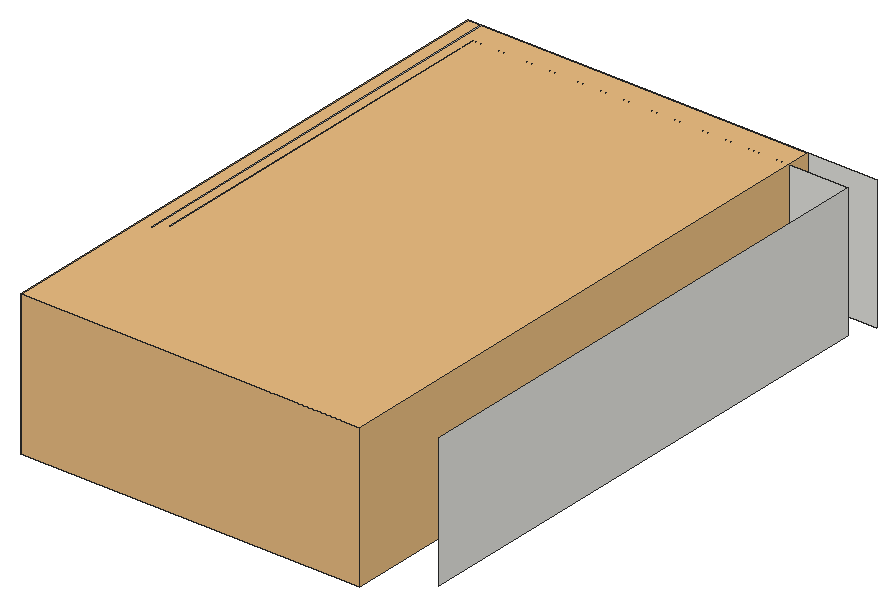
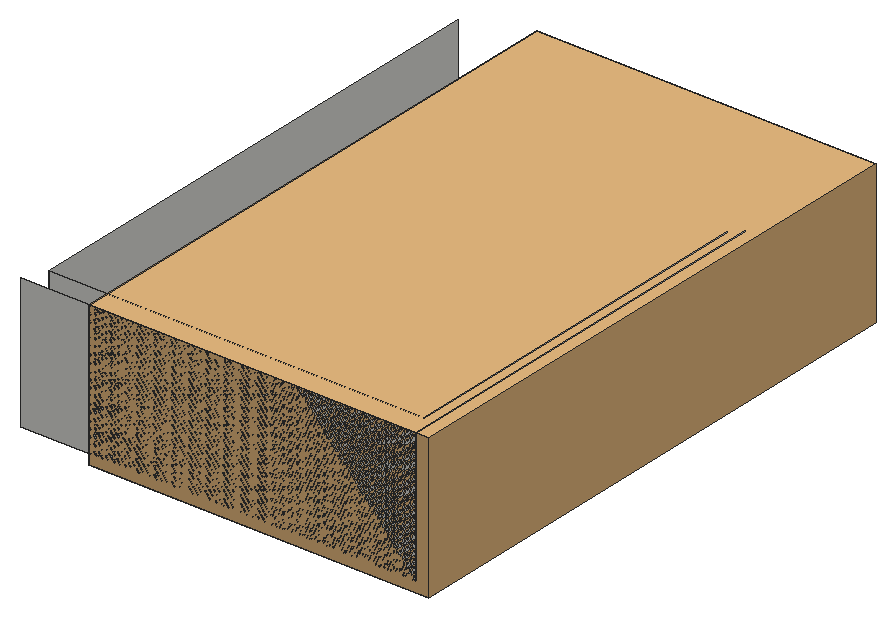
# SketchUp Ruby script. Lengths in inches.
U = 1.inch
M = Sketchup.active_model
def pt(a) = Geom::Point3d.new(a.map { |v| v * U })
def face(e, loops, mat)
  f = e.add_face(loops[0].map { |a| pt(a) })
  loops[1..].each { |l| e.add_face(l.map { |a| pt(a) }).erase! }
  f.material = f.back_material = mat if mat
  f
end
# faces: each face lists its corners as indices into pts; further lists are holes
def faces(e, pts, list, mat = nil) = list.each { |f| face(e, (f[0].is_a?(Array) ? f : [f]).map { |l| l.map { |i| pts[i] } }, mat) }
# xy, xz, yz: faces in a plane at the given z, y or x. An outline is a flat list of corners, or four numbers for a rectangle; further outlines are holes
def ring(l) = l.size == 4 ? [[l[0], l[1]], [l[2], l[1]], [l[2], l[3]], [l[0], l[3]]] : l.each_slice(2).to_a
def flat(e, list, mat, &to3) = list.each { |f| face(e, (f[0].is_a?(Array) ? f : [f]).map { |l| ring(l).map { |u, v| to3.(u, v) } }, mat) }
def xy(e, z, list, mat = nil) = flat(e, list, mat) { |x, y| [x, y, z] }
def xz(e, y, list, mat = nil) = flat(e, list, mat) { |x, z| [x, y, z] }
def yz(e, x, list, mat = nil) = flat(e, list, mat) { |y, z| [x, y, z] }
def lines(e, pts, list) = list.each { |a, b| e.add_line(pt(pts[a]), pt(pts[b])) }
# prism: a flat outline (further loops are holes) pulled along v
def prism(e, loops, v, mat = nil)
  f = face(e, loops, mat); d = Geom::Vector3d.new(v.map { |x| x * U })
  f.pushpull(f.normal.samedirection?(d) ? d.length : -d.length)
end
def box(e, o, s, mat = nil) = prism(e, [[o, [o[0] + s[0], o[1], o[2]], [o[0] + s[0], o[1] + s[1], o[2]], [o[0], o[1] + s[1], o[2]]]], [0, 0, s[2]], mat)
def at(x, y, z, deg = 0) = Geom::Transformation.translation(pt([x, y, z])) * Geom::Transformation.rotation(ORIGIN, Z_AXIS, deg.degrees)
def axes(o, x, y, z) = Geom::Transformation.new([*x, 0, *y, 0, *z, 0, *pt(o).to_a, 1])
def part(name) = M.definitions.add(name)
# library, detail: a bought-in or finely detailed component or shape, given as its bounding box
def library(name, o, s) = part(name).tap { |d| box(d.entities, o, s) }
def detail(e, o, s) = box(e.add_group.entities, o, s)
def put(e, d, t, mat = nil) = e.add_instance(d, t).tap { |i| i.material = mat if mat }
def group(e, t, mat = nil) = e.add_group.tap { |g| g.transformation = t; g.material = mat if mat }.entities
root = M.entities
M.materials.add("1122 AP 7994 PEACH ROSE").color = [254, 227, 201]
M.materials.add("[Quartz Light Grey]").color = [251, 251, 252]
c1 = library("Group\#12",[-2,-2,0],[309,506,129])
xy(root,152.82,[[40.86,300.07,40.7,300.09,40.55,300.11,40.47,300.12,40.39,300.14,40.32,300.15,40.16,300.19,40.09,300.22,40.01,300.24,39.8,300.33,39.72,300.36,39.65,300.4,39.58,300.43,39.52,300.47,39.38,300.55,39.32,300.6,39.25,300.64,38.95,300.89,38.89,300.95,38.84,301.01,38.79,301.0625,38.74,301.12,38.68,301.18,38.64,301.24,38.59,301.31,38.54,301.37,38.5,301.4375,38.46,301.5,38.34,301.71,38.28,301.85,38.24,301.92,38.22,302,38.1875,302.07,38.16,302.14,38.14,302.22,38.12,302.29,38.08,302.45,38.07,302.52,38.05,302.6,38.03,302.76,38.03,302.84,38.02,302.91,38.02,303.23,38.03,303.31,38.03,303.38,38.05,303.54,38.07,303.62,38.08,303.69,38.12,303.85,38.14,303.92,38.16,304,38.1875,304.07,38.22,304.15,38.24,304.22,38.28,304.29,38.34,304.43,38.46,304.64,38.5,304.7,38.54,304.77,38.59,304.83,38.64,304.9,38.68,304.96,38.74,305.02,38.84,305.14,38.95,305.25,39.25,305.5,39.32,305.54,39.38,305.59,39.52,305.67,39.58,305.71,39.65,305.74,39.72,305.78,39.8,305.8125,39.87,305.84,40.01,305.9,40.09,305.92,40.16,305.95,40.32,305.99,40.39,306.01,40.55,306.03,40.625,306.05,40.7,306.05,40.78,306.0625,40.86,306.07,41.17,306.07,41.25,306.0625,41.33,306.05,41.41,306.05,41.49,306.03,41.5625,306.02,41.64,306.01,41.72,305.99,41.79,305.97,41.87,305.95,41.94,305.92,42.02,305.9,42.16,305.84,42.24,305.8125,42.31,305.78,42.38,305.74,42.45,305.71,42.52,305.67,42.58,305.63,42.65,305.59,42.72,305.54,42.78,305.5,43.08,305.25,43.25,305.08,43.4,304.9,43.44,304.83,43.49,304.77,43.53,304.7,43.57,304.64,43.65,304.5,43.6875,304.43,43.72,304.36,43.76,304.29,43.82,304.15,43.84,304.07,43.87,304,43.89,303.92,43.91,303.85,43.95,303.69,43.97,303.62,44,303.38,44.01,303.31,44.01,303.23,44.02,303.15,44.02,302.99,44.01,302.91,44.01,302.84,43.97,302.52,43.95,302.45,43.91,302.29,43.89,302.22,43.87,302.14,43.84,302.07,43.82,302,43.79,301.92,43.76,301.85,43.72,301.78,43.6875,301.71,43.65,301.64,43.57,301.5,43.53,301.4375,43.49,301.37,43.44,301.31,43.4,301.24,43.3,301.12,43.25,301.0625,43.19,301.01,43.14,300.95,43.08,300.89,42.78,300.64,42.72,300.6,42.65,300.55,42.58,300.51,42.52,300.47,42.45,300.43,42.38,300.4,42.31,300.36,42.24,300.33,42.16,300.3,42.02,300.24,41.94,300.22,41.87,300.19,41.79,300.17,41.72,300.15,41.64,300.14,41.5625,300.12,41.49,300.11,41.17,300.07],[104.79,300.07,104.72,300.08,104.4,300.12,104.33,300.14,104.25,300.15,104.17,300.17,104.1,300.19,104.02,300.22,103.95,300.24,103.8,300.3,103.66,300.36,103.59,300.4,103.52,300.43,103.38,300.51,103.32,300.55,103.25,300.6,103.1875,300.64,103,300.79,102.94,300.84,102.83,300.95,102.78,301.01,102.72,301.0625,102.67,301.12,102.57,301.24,102.52,301.31,102.48,301.37,102.44,301.4375,102.39,301.5,102.31,301.64,102.28,301.71,102.24,301.78,102.18,301.92,102.15,302,102.1,302.14,102.07,302.22,102.05,302.29,102.03,302.37,102.02,302.45,102,302.52,101.96,302.84,101.96,302.91,101.95,302.99,101.95,303.15,101.96,303.23,101.96,303.31,101.97,303.38,102,303.62,102.02,303.69,102.03,303.77,102.05,303.85,102.07,303.92,102.1,304,102.125,304.07,102.15,304.15,102.24,304.36,102.28,304.43,102.31,304.5,102.39,304.64,102.44,304.7,102.48,304.77,102.52,304.83,102.57,304.9,102.72,305.08,102.94,305.3,103,305.35,103.1875,305.5,103.25,305.54,103.32,305.59,103.38,305.63,103.52,305.71,103.59,305.74,103.66,305.78,103.73,305.8125,103.8,305.84,103.95,305.9,104.02,305.92,104.1,305.95,104.17,305.97,104.33,306.01,104.4,306.02,104.48,306.03,104.56,306.05,104.64,306.05,104.72,306.0625,104.79,306.07,105.11,306.07,105.1875,306.0625,105.26,306.05,105.34,306.05,105.42,306.03,105.5,306.02,105.57,306.01,105.73,305.97,105.8,305.95,105.88,305.92,105.95,305.9,106.03,305.87,106.1,305.84,106.17,305.8125,106.24,305.78,106.3125,305.74,106.38,305.71,106.59,305.59,106.65,305.54,106.71,305.5,106.78,305.45,107.02,305.25,107.07,305.19,107.13,305.14,107.33,304.9,107.38,304.83,107.42,304.77,107.47,304.7,107.51,304.64,107.59,304.5,107.66,304.36,107.75,304.15,107.78,304.07,107.8,304,107.83,303.92,107.85,303.85,107.89,303.69,107.9,303.62,107.91,303.54,107.93,303.46,107.93,303.38,107.94,303.31,107.95,303.23,107.95,302.91,107.94,302.84,107.93,302.76,107.93,302.68,107.91,302.6,107.9,302.52,107.89,302.45,107.85,302.29,107.83,302.22,107.8,302.14,107.78,302.07,107.75,302,107.72,301.92,107.66,301.78,107.59,301.64,107.51,301.5,107.47,301.4375,107.42,301.37,107.38,301.31,107.33,301.24,107.23,301.12,107.18,301.0625,107.13,301.01,107.07,300.95,107.02,300.89,106.78,300.69,106.71,300.64,106.65,300.6,106.59,300.55,106.38,300.43,106.3125,300.4,106.24,300.36,106.03,300.27,105.95,300.24,105.88,300.22,105.8,300.19,105.73,300.17,105.65,300.15,105.57,300.14,105.5,300.12,105.26,300.09,105.1875,300.08,105.11,300.07]],"1122 AP 7994 PEACH ROSE")
xz(root,306.05,[[104.56,149.82,104.64,152.82],[105.26,149.82,105.34,152.82]],"1122 AP 7994 PEACH ROSE")
xz(root,306.07,[[104.79,149.82,104.87,152.82],[104.87,149.82,104.95,152.82],[104.95,149.82,105.03,152.82],[105.03,149.82,105.11,152.82]],"1122 AP 7994 PEACH ROSE")
xz(root,624,[[18,158.82,357,278.82]])
xz(root,645,[[9,158.82,366,278.82]])
yz(root,9,[[273,158.82,645,278.82]])
yz(root,18,[[282,158.82,624,278.82]])
yz(root,101.95,[[302.99,149.82,303.07,152.82],[303.07,149.82,303.15,152.82]],"1122 AP 7994 PEACH ROSE")
yz(root,101.96,[[302.84,149.82,302.91,152.82],[303.23,149.82,303.31,152.82]],"1122 AP 7994 PEACH ROSE")
yz(root,107.93,[[302.68,149.82,302.76,152.82],[303.38,149.82,303.46,152.82]],"1122 AP 7994 PEACH ROSE")
yz(root,107.95,[[302.91,149.82,302.99,152.82],[302.99,149.82,303.07,152.82],[303.07,149.82,303.15,152.82],[303.15,149.82,303.23,152.82]],"1122 AP 7994 PEACH ROSE")
yz(root,357,[[162,158.82,624,278.82]])
p = [[104.4,300.12,149.82],[104.33,300.14,149.82],[104.33,300.14,152.82],[104.4,300.12,152.82],[104.25,300.15,149.82],[104.25,300.15,152.82],
  [104.48,300.11,149.82],[104.48,300.11,152.82],[105.57,300.14,149.82],[105.5,300.12,149.82],[105.5,300.12,152.82],[105.57,300.14,152.82],
  [105.65,300.15,149.82],[105.65,300.15,152.82],[104.02,300.22,149.82],[103.95,300.24,149.82],[103.95,300.24,152.82],[104.02,300.22,152.82],
  [103.875,300.27,149.82],[103.875,300.27,152.82],[104.1,300.19,149.82],[104.1,300.19,152.82],[104.17,300.17,149.82],[104.17,300.17,152.82],
  [105.73,300.17,149.82],[105.73,300.17,152.82],[105.8,300.19,149.82],[105.8,300.19,152.82],[105.88,300.22,149.82],[105.88,300.22,152.82],
  [105.95,300.24,149.82],[105.95,300.24,152.82],[106.03,300.27,149.82],[106.03,300.27,152.82],[103.8,300.3,149.82],[103.73,300.33,149.82],
  [103.73,300.33,152.82],[103.8,300.3,152.82],[103.66,300.36,149.82],[103.66,300.36,152.82],[106.1,300.3,149.82],[106.1,300.3,152.82],
  [106.17,300.33,149.82],[106.17,300.33,152.82],[106.24,300.36,149.82],[106.24,300.36,152.82],[103.59,300.4,149.82],[103.52,300.43,149.82],
  [103.52,300.43,152.82],[103.59,300.4,152.82],[103.45,300.47,149.82],[103.45,300.47,152.82],[106.3125,300.4,149.82],[106.3125,300.4,152.82],
  [106.38,300.43,149.82],[106.38,300.43,152.82],[106.45,300.47,149.82],[106.45,300.47,152.82],[103.38,300.51,149.82],[103.32,300.55,149.82],
  [103.32,300.55,152.82],[103.38,300.51,152.82],[106.52,300.51,149.82],[106.52,300.51,152.82],[106.59,300.55,149.82],[106.59,300.55,152.82],
  [103.1875,300.64,149.82],[103.125,300.69,149.82],[103.125,300.69,152.82],[103.1875,300.64,152.82],[103.25,300.6,149.82],[103.25,300.6,152.82],
  [106.65,300.6,149.82],[106.65,300.6,152.82],[106.71,300.64,149.82],[106.71,300.64,152.82],[106.78,300.69,149.82],[106.78,300.69,152.82],
  [103.0625,300.74,149.82],[103,300.79,149.82],[103,300.79,152.82],[103.0625,300.74,152.82],[106.84,300.74,149.82],[106.84,300.74,152.82],
  [106.9,300.79,149.82],[106.9,300.79,152.82],[102.94,300.84,149.82],[102.94,300.84,152.82],[102.89,300.89,149.82],[102.89,300.89,152.82],
  [106.96,300.84,149.82],[106.96,300.84,152.82],[107.02,300.89,149.82],[107.02,300.89,152.82],[102.83,300.95,149.82],[102.83,300.95,152.82],
  [102.78,301.01,149.82],[102.78,301.01,152.82],[107.07,300.95,149.82],[107.07,300.95,152.82],[107.13,301.01,149.82],[107.13,301.01,152.82],
  [102.72,301.0625,149.82],[102.72,301.0625,152.82],[107.18,301.0625,149.82],[107.18,301.0625,152.82],[102.67,301.12,149.82],[102.62,301.18,149.82],
  [102.62,301.18,152.82],[102.67,301.12,152.82],[107.23,301.12,149.82],[107.23,301.12,152.82],[107.28,301.18,149.82],[107.28,301.18,152.82],
  [102.57,301.24,149.82],[102.52,301.31,149.82],[102.52,301.31,152.82],[102.57,301.24,152.82],[107.33,301.24,149.82],[107.33,301.24,152.82],
  [107.38,301.31,149.82],[107.38,301.31,152.82],[102.48,301.37,149.82],[102.48,301.37,152.82],[107.42,301.37,149.82],[107.42,301.37,152.82],
  [102.44,301.4375,149.82],[102.44,301.4375,152.82],[102.39,301.5,149.82],[102.39,301.5,152.82],[107.47,301.4375,149.82],[107.47,301.4375,152.82],
  [107.51,301.5,149.82],[107.51,301.5,152.82],[102.35,301.57,149.82],[102.35,301.57,152.82],[107.55,301.57,149.82],[107.55,301.57,152.82],
  [102.31,301.64,149.82],[102.31,301.64,152.82],[102.28,301.71,149.82],[102.28,301.71,152.82],[107.59,301.64,149.82],[107.59,301.64,152.82],
  [107.625,301.71,149.82],[107.625,301.71,152.82],[102.24,301.78,149.82],[102.24,301.78,152.82],[107.66,301.78,149.82],[107.66,301.78,152.82],
  [102.21,301.85,149.82],[102.21,301.85,152.82],[107.69,301.85,149.82],[107.69,301.85,152.82],[102.18,301.92,149.82],[102.18,301.92,152.82],
  [102.15,302,149.82],[102.15,302,152.82],[107.72,301.92,149.82],[107.72,301.92,152.82],[107.75,302,149.82],[107.75,302,152.82],
  [102.125,302.07,149.82],[102.125,302.07,152.82],[107.78,302.07,149.82],[107.78,302.07,152.82],[102.1,302.14,149.82],[102.1,302.14,152.82],
  [102.07,302.22,149.82],[102.07,302.22,152.82],[107.8,302.14,149.82],[107.8,302.14,152.82],[107.83,302.22,149.82],[107.83,302.22,152.82],
  [102.05,302.29,149.82],[102.05,302.29,152.82],[107.85,302.29,149.82],[107.85,302.29,152.82],[102.03,302.37,149.82],[102.03,302.37,152.82],
  [107.87,302.37,149.82],[107.87,302.37,152.82],[102.02,302.45,149.82],[102.02,302.45,152.82],[102,302.52,149.82],[102,302.52,152.82],
  [107.89,302.45,149.82],[107.89,302.45,152.82],[107.9,302.52,149.82],[107.9,302.52,152.82],[101.99,302.6,149.82],[101.99,302.6,152.82],
  [107.91,302.6,149.82],[107.91,302.6,152.82],[101.98,302.68,149.82],[101.98,302.68,152.82],[107.93,302.68,149.82],[107.93,302.68,152.82],
  [101.97,302.76,149.82],[101.97,302.76,152.82],[101.96,302.84,149.82],[101.96,302.84,152.82],[107.94,302.84,149.82],[107.93,302.76,149.82],
  [107.93,302.76,152.82],[107.94,302.84,152.82],[107.95,302.91,149.82],[107.95,302.91,152.82],[101.96,302.91,149.82],[101.95,302.99,149.82],
  [101.95,302.99,152.82],[101.96,302.91,152.82],[101.95,303.15,149.82],[101.96,303.23,149.82],[101.96,303.23,152.82],[101.95,303.15,152.82],
  [107.94,303.31,149.82],[107.95,303.23,149.82],[107.95,303.23,152.82],[107.94,303.31,152.82],[101.96,303.31,149.82],[101.97,303.38,149.82],
  [101.97,303.38,152.82],[101.96,303.31,152.82],[107.93,303.38,149.82],[107.93,303.38,152.82],[101.98,303.46,149.82],[101.98,303.46,152.82],
  [101.99,303.54,149.82],[101.99,303.54,152.82],[102,303.62,149.82],[102,303.62,152.82],[107.91,303.54,149.82],[107.93,303.46,149.82],
  [107.93,303.46,152.82],[107.91,303.54,152.82],[107.9,303.62,149.82],[107.9,303.62,152.82],[102.02,303.69,149.82],[102.02,303.69,152.82],
  [107.89,303.69,149.82],[107.89,303.69,152.82],[102.03,303.77,149.82],[102.03,303.77,152.82],[107.87,303.77,149.82],[107.87,303.77,152.82],
  [102.05,303.85,149.82],[102.05,303.85,152.82],[102.07,303.92,149.82],[102.07,303.92,152.82],[107.85,303.85,149.82],[107.85,303.85,152.82],
  [107.83,303.92,149.82],[107.83,303.92,152.82],[102.1,304,149.82],[102.1,304,152.82],[107.8,304,149.82],[107.8,304,152.82],
  [102.125,304.07,149.82],[102.125,304.07,152.82],[107.78,304.07,149.82],[107.78,304.07,152.82],[102.15,304.15,149.82],[102.15,304.15,152.82],
  [102.18,304.22,149.82],[102.18,304.22,152.82],[107.72,304.22,149.82],[107.75,304.15,149.82],[107.75,304.15,152.82],[107.72,304.22,152.82],
  [102.21,304.29,149.82],[102.21,304.29,152.82],[107.69,304.29,149.82],[107.69,304.29,152.82],[102.24,304.36,149.82],[102.24,304.36,152.82],
  [107.66,304.36,149.82],[107.66,304.36,152.82],[102.28,304.43,149.82],[102.28,304.43,152.82],[102.31,304.5,149.82],[102.31,304.5,152.82],
  [107.625,304.43,149.82],[107.625,304.43,152.82],[107.59,304.5,149.82],[107.59,304.5,152.82],[102.35,304.57,149.82],[102.35,304.57,152.82],
  [107.55,304.57,149.82],[107.55,304.57,152.82],[102.39,304.64,149.82],[102.39,304.64,152.82],[102.44,304.7,149.82],[102.44,304.7,152.82],
  [107.51,304.64,149.82],[107.51,304.64,152.82],[107.47,304.7,149.82],[107.47,304.7,152.82],[102.48,304.77,149.82],[102.48,304.77,152.82],
  [107.42,304.77,149.82],[107.42,304.77,152.82],[102.52,304.83,149.82],[102.52,304.83,152.82],[102.57,304.9,149.82],[102.57,304.9,152.82],
  [107.33,304.9,149.82],[107.38,304.83,149.82],[107.38,304.83,152.82],[107.33,304.9,152.82],[102.62,304.96,149.82],[102.62,304.96,152.82],
  [107.28,304.96,149.82],[107.28,304.96,152.82],[102.67,305.02,149.82],[102.67,305.02,152.82],[102.72,305.08,149.82],[102.72,305.08,152.82],
  [107.23,305.02,149.82],[107.23,305.02,152.82],[107.18,305.08,149.82],[107.18,305.08,152.82],[102.78,305.14,149.82],[102.78,305.14,152.82],
  [102.83,305.19,149.82],[102.83,305.19,152.82],[107.13,305.14,149.82],[107.13,305.14,152.82],[107.07,305.19,149.82],[107.07,305.19,152.82],
  [102.89,305.25,149.82],[102.89,305.25,152.82],[102.94,305.3,149.82],[102.94,305.3,152.82],[107.02,305.25,149.82],[107.02,305.25,152.82],
  [106.96,305.3,149.82],[106.96,305.3,152.82],[103,305.35,149.82],[103,305.35,152.82],[106.9,305.35,149.82],[106.9,305.35,152.82],
  [103.0625,305.4,149.82],[103.0625,305.4,152.82],[103.125,305.45,149.82],[103.125,305.45,152.82],[106.84,305.4,149.82],[106.84,305.4,152.82],
  [106.78,305.45,149.82],[106.78,305.45,152.82],[103.1875,305.5,149.82],[103.1875,305.5,152.82],[103.25,305.54,149.82],[103.25,305.54,152.82],
  [103.32,305.59,149.82],[103.32,305.59,152.82],[106.59,305.59,149.82],[106.65,305.54,149.82],[106.65,305.54,152.82],[106.59,305.59,152.82],
  [106.71,305.5,149.82],[106.71,305.5,152.82],[103.38,305.63,149.82],[103.38,305.63,152.82],[103.45,305.67,149.82],[103.45,305.67,152.82],
  [106.52,305.63,149.82],[106.52,305.63,152.82],[106.45,305.67,149.82],[106.45,305.67,152.82],[103.52,305.71,149.82],[103.52,305.71,152.82],
  [103.59,305.74,149.82],[103.59,305.74,152.82],[103.66,305.78,149.82],[103.66,305.78,152.82],[106.24,305.78,149.82],[106.3125,305.74,149.82],
  [106.3125,305.74,152.82],[106.24,305.78,152.82],[106.38,305.71,149.82],[106.38,305.71,152.82],[103.73,305.8125,149.82],[103.73,305.8125,152.82],
  [103.8,305.84,149.82],[103.8,305.84,152.82],[103.875,305.87,149.82],[103.875,305.87,152.82],[106.03,305.87,149.82],[106.1,305.84,149.82],
  [106.1,305.84,152.82],[106.03,305.87,152.82],[106.17,305.8125,149.82],[106.17,305.8125,152.82],[103.95,305.9,149.82],[103.95,305.9,152.82],
  [104.02,305.92,149.82],[104.02,305.92,152.82],[104.1,305.95,149.82],[104.1,305.95,152.82],[104.17,305.97,149.82],[104.17,305.97,152.82],
  [105.73,305.97,149.82],[105.8,305.95,149.82],[105.8,305.95,152.82],[105.73,305.97,152.82],[105.88,305.92,149.82],[105.88,305.92,152.82],
  [105.95,305.9,149.82],[105.95,305.9,152.82],[104.25,305.99,149.82],[104.25,305.99,152.82],[104.33,306.01,149.82],[104.33,306.01,152.82],
  [104.4,306.02,149.82],[104.4,306.02,152.82],[104.48,306.03,149.82],[104.48,306.03,152.82],[104.56,306.05,149.82],[104.56,306.05,152.82],
  [105.34,306.05,149.82],[105.42,306.03,149.82],[105.42,306.03,152.82],[105.34,306.05,152.82],[105.5,306.02,149.82],[105.5,306.02,152.82],
  [105.57,306.01,149.82],[105.57,306.01,152.82],[105.65,305.99,149.82],[105.65,305.99,152.82],[104.64,306.05,149.82],[104.72,306.0625,149.82],
  [104.72,306.0625,152.82],[104.64,306.05,152.82],[104.79,306.07,149.82],[104.79,306.07,152.82],[105.11,306.07,149.82],[105.1875,306.0625,149.82],
  [105.1875,306.0625,152.82],[105.11,306.07,152.82],[105.26,306.05,149.82],[105.26,306.05,152.82]]
faces(root,p,[[0,1,2,3],[1,4,5,2],[6,0,3,7],[8,9,10,11],[12,8,11,13],[14,15,16,17],[15,18,19,16],[20,14,17,21],
  [22,20,21,23],[4,22,23,5],[24,12,13,25],[26,24,25,27],[28,26,27,29],[30,28,29,31],[32,30,31,33],[34,35,36,37],
  [35,38,39,36],[18,34,37,19],[40,32,33,41],[42,40,41,43],[44,42,43,45],[46,47,48,49],[47,50,51,48],[38,46,49,39],
  [52,44,45,53],[54,52,53,55],[56,54,55,57],[58,59,60,61],[50,58,61,51],[62,56,57,63],[64,62,63,65],[66,67,68,69],
  [70,66,69,71],[59,70,71,60],[72,64,65,73],[74,72,73,75],[76,74,75,77],[78,79,80,81],[67,78,81,68],[82,76,77,83],
  [84,82,83,85],[79,86,87,80],[86,88,89,87],[90,84,85,91],[92,90,91,93],[88,94,95,89],[94,96,97,95],[98,92,93,99],
  [100,98,99,101],[96,102,103,97],[104,100,101,105],[106,107,108,109],[102,106,109,103],[110,104,105,111],[112,110,111,113],[114,115,116,117],
  [107,114,117,108],[118,112,113,119],[120,118,119,121],[115,122,123,116],[124,120,121,125],[122,126,127,123],[126,128,129,127],[130,124,125,131],
  [132,130,131,133],[128,134,135,129],[136,132,133,137],[134,138,139,135],[138,140,141,139],[142,136,137,143],[144,142,143,145],[140,146,147,141],
  [148,144,145,149],[146,150,151,147],[152,148,149,153],[150,154,155,151],[154,156,157,155],[158,152,153,159],[160,158,159,161],[156,162,163,157],
  [164,160,161,165],[162,166,167,163],[166,168,169,167],[170,164,165,171],[172,170,171,173],[168,174,175,169],[176,172,173,177],[174,178,179,175],
  [180,176,177,181],[178,182,183,179],[182,184,185,183],[186,180,181,187],[188,186,187,189],[184,190,191,185],[192,188,189,193],[190,194,195,191],
  [196,192,193,197],[194,198,199,195],[198,200,201,199],[202,203,204,205],[206,202,205,207],[208,209,210,211],[212,213,214,215],[216,217,218,219],
  [220,221,222,223],[224,216,219,225],[221,226,227,222],[226,228,229,227],[228,230,231,229],[232,233,234,235],[236,232,235,237],[230,238,239,231],
  [240,236,237,241],[238,242,243,239],[244,240,241,245],[242,246,247,243],[246,248,249,247],[250,244,245,251],[252,250,251,253],[248,254,255,249],
  [256,252,253,257],[254,258,259,255],[260,256,257,261],[258,262,263,259],[262,264,265,263],[266,267,268,269],[267,260,261,268],[264,270,271,265],
  [272,266,269,273],[270,274,275,271],[276,272,273,277],[274,278,279,275],[278,280,281,279],[282,276,277,283],[284,282,283,285],[280,286,287,281],
  [288,284,285,289],[286,290,291,287],[290,292,293,291],[294,288,289,295],[296,294,295,297],[292,298,299,293],[300,296,297,301],[298,302,303,299],
  [302,304,305,303],[306,307,308,309],[307,300,301,308],[304,310,311,305],[312,306,309,313],[310,314,315,311],[314,316,317,315],[318,312,313,319],
  [320,318,319,321],[316,322,323,317],[322,324,325,323],[326,320,321,327],[328,326,327,329],[324,330,331,325],[330,332,333,331],[334,328,329,335],
  [336,334,335,337],[332,338,339,333],[340,336,337,341],[338,342,343,339],[342,344,345,343],[346,340,341,347],[348,346,347,349],[344,350,351,345],
  [350,352,353,351],[352,354,355,353],[356,357,358,359],[360,348,349,361],[357,360,361,358],[354,362,363,355],[362,364,365,363],[366,356,359,367],
  [368,366,367,369],[364,370,371,365],[370,372,373,371],[372,374,375,373],[376,377,378,379],[377,380,381,378],[380,368,369,381],[374,382,383,375],
  [382,384,385,383],[384,386,387,385],[388,389,390,391],[389,392,393,390],[392,376,379,393],[386,394,395,387],[394,396,397,395],[396,398,399,397],
  [398,400,401,399],[402,403,404,405],[403,406,407,404],[406,408,409,407],[408,388,391,409],[400,410,411,401],[410,412,413,411],[412,414,415,413],
  [414,416,417,415],[416,418,419,417],[420,421,422,423],[421,424,425,422],[424,426,427,425],[426,428,429,427],[428,402,405,429],[430,431,432,433],
  [431,434,435,432],[436,437,438,439],[437,440,441,438]],"1122 AP 7994 PEACH ROSE")
put(root,c1,axes([-0.85,141,149.82],[0.993,0,0],[0,1,0],[0,0,1]),"[Quartz Light Grey]")
